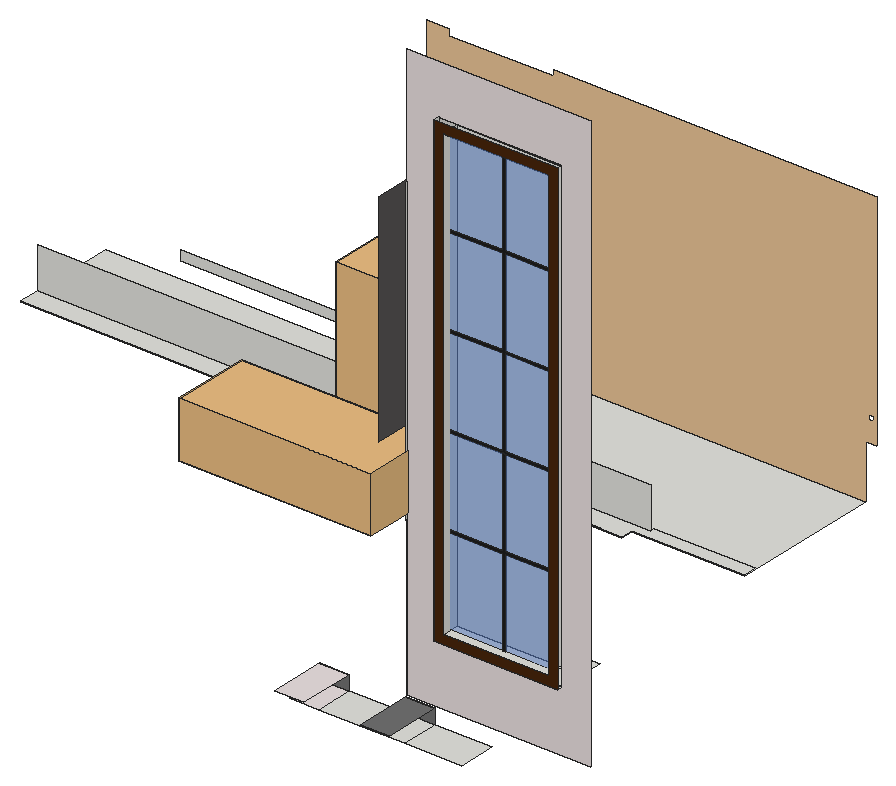
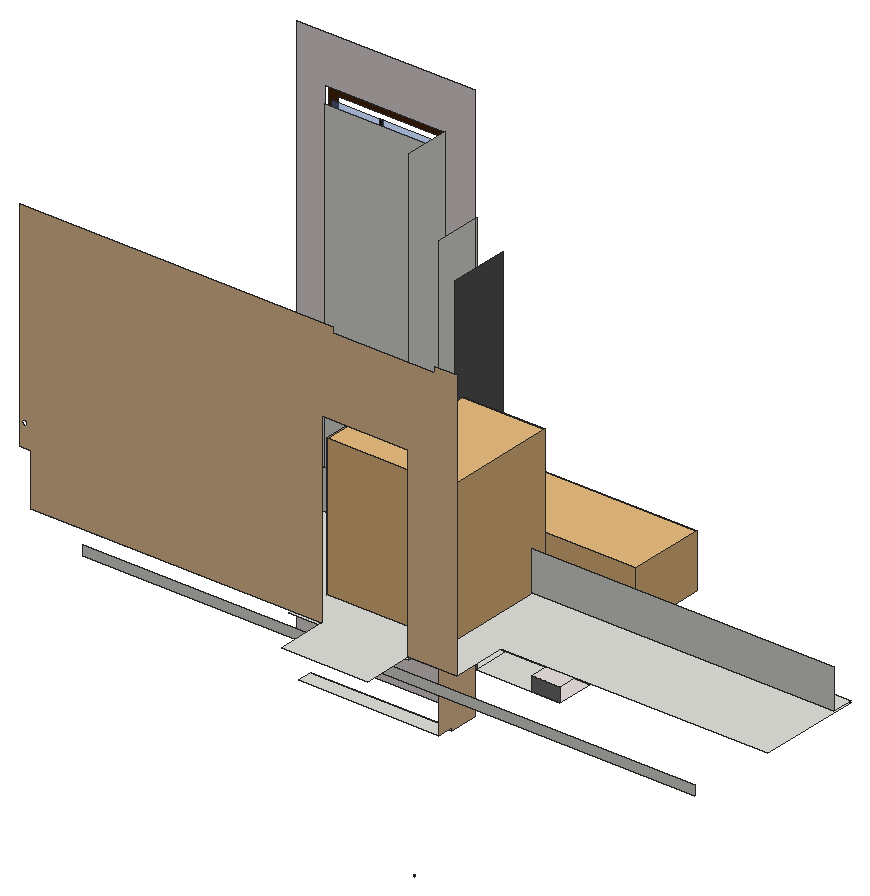
# SketchUp Ruby script. Lengths in inches.
U = 1.inch
M = Sketchup.active_model
def pt(a) = Geom::Point3d.new(a.map { |v| v * U })
def face(e, loops, mat)
  f = e.add_face(loops[0].map { |a| pt(a) })
  loops[1..].each { |l| e.add_face(l.map { |a| pt(a) }).erase! }
  f.material = f.back_material = mat if mat
  f
end
# faces: each face lists its corners as indices into pts; further lists are holes
def faces(e, pts, list, mat = nil) = list.each { |f| face(e, (f[0].is_a?(Array) ? f : [f]).map { |l| l.map { |i| pts[i] } }, mat) }
# xy, xz, yz: faces in a plane at the given z, y or x. An outline is a flat list of corners, or four numbers for a rectangle; further outlines are holes
def ring(l) = l.size == 4 ? [[l[0], l[1]], [l[2], l[1]], [l[2], l[3]], [l[0], l[3]]] : l.each_slice(2).to_a
def flat(e, list, mat, &to3) = list.each { |f| face(e, (f[0].is_a?(Array) ? f : [f]).map { |l| ring(l).map { |u, v| to3.(u, v) } }, mat) }
def xy(e, z, list, mat = nil) = flat(e, list, mat) { |x, y| [x, y, z] }
def xz(e, y, list, mat = nil) = flat(e, list, mat) { |x, z| [x, y, z] }
def yz(e, x, list, mat = nil) = flat(e, list, mat) { |y, z| [x, y, z] }
def lines(e, pts, list) = list.each { |a, b| e.add_line(pt(pts[a]), pt(pts[b])) }
# prism: a flat outline (further loops are holes) pulled along v
def prism(e, loops, v, mat = nil)
  f = face(e, loops, mat); d = Geom::Vector3d.new(v.map { |x| x * U })
  f.pushpull(f.normal.samedirection?(d) ? d.length : -d.length)
end
def box(e, o, s, mat = nil) = prism(e, [[o, [o[0] + s[0], o[1], o[2]], [o[0] + s[0], o[1] + s[1], o[2]], [o[0], o[1] + s[1], o[2]]]], [0, 0, s[2]], mat)
def at(x, y, z, deg = 0) = Geom::Transformation.translation(pt([x, y, z])) * Geom::Transformation.rotation(ORIGIN, Z_AXIS, deg.degrees)
def axes(o, x, y, z) = Geom::Transformation.new([*x, 0, *y, 0, *z, 0, *pt(o).to_a, 1])
def part(name) = M.definitions.add(name)
# library, detail: a bought-in or finely detailed component or shape, given as its bounding box
def library(name, o, s) = part(name).tap { |d| box(d.entities, o, s) }
def detail(e, o, s) = box(e.add_group.entities, o, s)
def put(e, d, t, mat = nil) = e.add_instance(d, t).tap { |i| i.material = mat if mat }
def group(e, t, mat = nil) = e.add_group.tap { |g| g.transformation = t; g.material = mat if mat }.entities
root = M.entities
M.materials.add("Generic\#1").color = [72, 38, 12]
M.materials.add("Generic\#2").color = [87, 84, 84]
M.materials.add("Generic\#4").color = [113, 113, 113]
M.materials.add("Generic\#8").color = [235, 197, 151]
M.materials.add("Generic\#9").color = [233, 223, 223]
M.materials.add("Material \#1").color = [140, 140, 140]
M.materials.add("[Color M08]").color = [30, 30, 30]
M.materials.add("[Translucent Glass Blue]").color = [100, 149, 237]
M.materials["[Translucent Glass Blue]"].alpha = 0.5
M.materials.add("[Translucent Glass Dark Green]").color = [62, 91, 5]
M.materials["[Translucent Glass Dark Green]"].alpha = 0.5
c1 = library("Plante \#58",[-0.43,-1.58,0],[20.84,18.06,17.59])
c2 = library("Group3\#1",[-238.15,54.18,0],[46.4,43.96,56.68])
xy(root,52.25,[[394.85,120.9375,454.48,127.4375]])
xy(root,56.4375,[[384.77,75.375,408.21,90.9375],[408.21,75.375,420.15,90.9375],[420.15,75.375,443.58,90.9375]])
xy(root,56.4375,[[372.83,75.375,384.77,90.9375]],"Generic\#9")
xy(root,62.5,[[408.21,67.75,420.15,90.9375]],"Generic\#4")
xy(root,62.5,[[372.83,67.75,384.77,90.9375]],"Generic\#9")
xy(root,76.26,[[407.84,106.0625,458.64,108.375],[407.84,108.375,458.64,127.4375]])
xy(root,80.07,[[411.65,106.0625,454.83,113.125]])
xy(root,126,[[220.54,127.4375,467.91,127.4375,467.91,132.5625,514.25,132.5625,514.25,194.75,390.67,194.75,390.67,216.25,354.24,216.25,354.24,194.75,333.65,194.75,333.65,171.4375,220.54,171.4375]])
xy(root,126.47,[[220.54,127.4375,220.54,136.1875,472.76,136.1875,472.76,138,514.25,138,514.25,132.5625,467.91,132.5625,467.91,127.4375]])
xz(root,90.9375,[[372.83,56.4375,384.77,62.5],[408.21,56.4375,420.15,62.5]],"Generic\#4")
xz(root,106.0625,[[[407.84,76.26,458.64,268.37],[411.65,80.07,454.83,264.56]]],"Generic\#1")
xz(root,108.375,[[[394.85,51,470.29,288.79],[407.84,76.26,458.64,268.37]]],"Generic\#9")
xz(root,113.125,[[411.65,80.07,454.83,264.56]])
xz(root,120.9375,[[394.85,51,454.48,52.25]])
xz(root,127.4375,[[394.85,126,407.84,126.47],[407.84,126,458.64,126.47],[383.85,126.47,394.85,143.28],[394.85,126.47,407.84,143.28]])
xz(root,136.1875,[[220.54,126.47,472.76,143.28]])
xz(root,194.75,[[[333.65,126,354.24,126,354.24,204.625,390.67,204.625,390.67,126,514.25,126,514.25,148.0625,518.6875,148.0625,518.6875,240,385.91,240,385.91,237.6875,342.98,237.6875,342.98,240,333.65,240],[516.7,156.58,516.42,156.62,516.15,156.73,515.92,156.91,515.75,157.14,515.63,157.4,515.6,157.69,515.63,157.98,515.75,158.24,515.92,158.47,516.15,158.65,516.42,158.76,516.7,158.8,516.99,158.76,517.26,158.65,517.49,158.47,517.66,158.24,517.77,157.98,517.8125,157.69,517.77,157.4,517.66,157.14,517.49,156.91,517.26,156.73,516.99,156.62]]],"Generic\#8")
xz(root,194.8125,[[232.6,115.8125,491.875,120]])
xz(root,199.31,[[347.91,46.81,347.9,46.82,347.9375,46.84],[347.91,46.81,347.9375,46.84,347.95,46.83],[347.95,46.83,347.9375,46.84,347.97,46.86],[347.95,46.83,347.97,46.86,347.98,46.85],[347.98,46.85,347.97,46.86,348,46.89],
  [347.98,46.85,348,46.89,348.01,46.88],[348.01,46.88,348,46.89,348.02,46.92],[347.95,47.25,347.9,47.26,347.91,47.27],[347.9,47.26,347.86,47.27,347.91,47.27],[347.86,47.27,347.82,47.28,347.87,47.28],
  [347.86,47.27,347.87,47.28,347.91,47.27],[347.82,47.28,347.82,47.29,347.87,47.28],[348.29,47.3125,348.18,47.375,348.1875,47.39],[348.18,47.375,348.07,47.43,348.1875,47.39],[348.1875,47.39,348.07,47.43,348.08,47.44],
  [347.82,47.47,347.82,47.49,347.95,47.47]],"Material \#1")
yz(root,383.85,[[[107.5625,126.47,107.5625,231,133.125,231,133.125,143.28,127.4375,143.28,127.4375,126.47],[128.02,155.04,130.65,156.97],[131.35,150.72,131.35,151.04,131.36,151.16,130.82,151.1875,130.82,151.0625,130.82,151.1875,130.19,151.1875,130.19,150.75,130.82,150.75],[131.35,148.72,131.35,149.04,131.36,149.16,130.82,149.1875,130.82,149.0625,130.82,149.1875,130.19,149.1875,130.19,148.75,130.82,148.75],[131.35,152.72,131.35,153.04,131.36,153.16,130.82,153.1875,130.82,153.0625,130.82,153.1875,130.19,153.1875,130.19,152.75,130.82,152.75]]],"Generic\#2")
yz(root,394.85,[[107.5625,115.8125,108.375,240],[108.375,115.8125,127.4375,240]])
yz(root,394.85,[[108.375,51,108.375,115.8125,127.4375,115.8125,127.4375,52.25,120.9375,52.25,120.9375,51]],"Generic\#8")
yz(root,407.84,[[106.0625,76.26,108.375,268.37],[108.375,76.26,127.4375,268.37]])
yz(root,411.65,[[106.0625,80.07,113.125,264.56]])
put(root,c1,axes([317.9,92.3125,117.94],[3.7878,0,0],[0,1.78,0],[0,0,1.3]))
put(root,c2,axes([617.68,67.89,121.28],[1.12793,0,0],[0,1.12793,0],[0,0,1.12793]))
g1 = group(root,at(411.65,109.5625,80.07),"[Translucent Glass Dark Green]")
xz(g1,0,[[21.59,0,22.79,0,22.79,35.86,43.18,35.86,43.18,36.9,22.79,36.9,22.79,72.76,21.59,72.76,21.59,36.9,0,36.9,0,35.86,21.59,35.86],[0,72.76,43.18,72.76,43.18,73.8,22.79,73.8,22.79,109.66,43.18,109.66,43.18,110.7,22.79,110.7,22.79,146.55,43.18,146.55,43.18,147.59,22.79,147.59,22.79,184.49,21.59,184.49,21.59,147.59,0,147.59,0,146.55,21.59,146.55,21.59,110.7,0,110.7,0,109.66,21.59,109.66,21.59,73.8,0,73.8]],"[Color M08]")
xz(g1,0,[[0,0,21.59,35.86],[22.79,0,43.18,35.86],[0,36.9,21.59,72.76],[22.79,36.9,43.18,72.76],[0,73.8,21.59,109.66],
  [22.79,73.8,43.18,109.66],[0,110.7,21.59,146.55],[22.79,110.7,43.18,146.55],[0,147.59,21.59,184.49],[22.79,147.59,43.18,184.49]],"[Translucent Glass Blue]")
